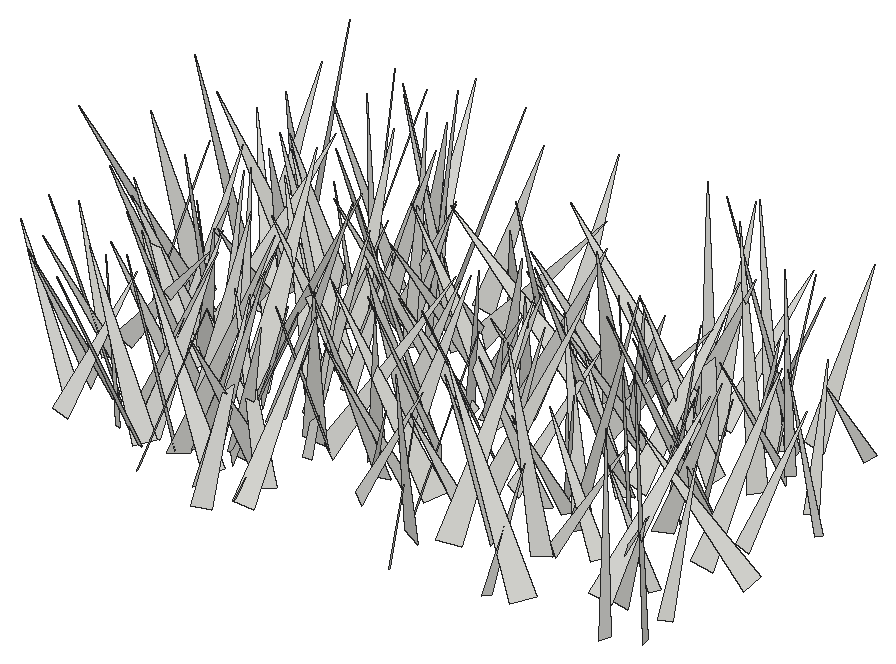
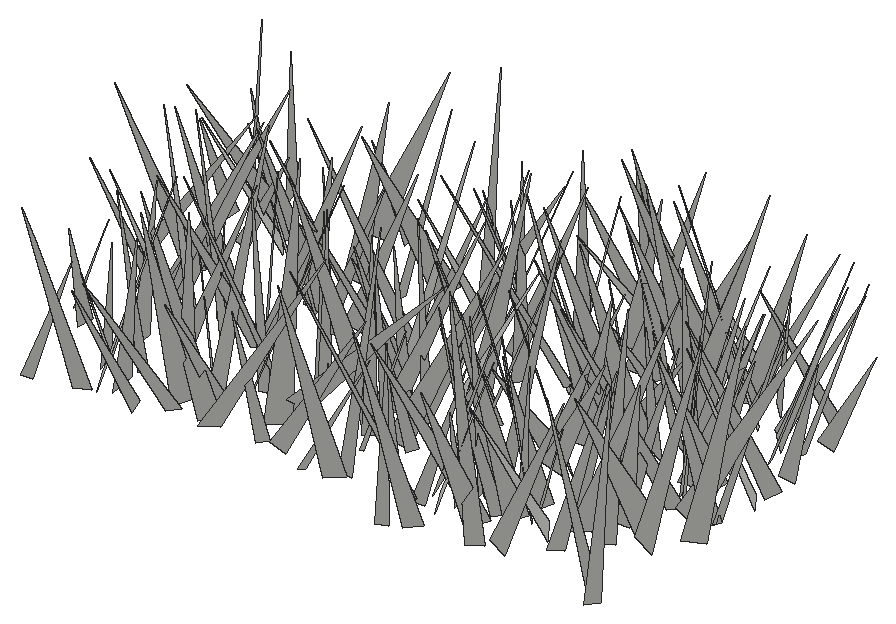
# SketchUp Ruby script. Lengths in inches.
U = 1.inch
M = Sketchup.active_model
def pt(a) = Geom::Point3d.new(a.map { |v| v * U })
def face(e, loops, mat)
  f = e.add_face(loops[0].map { |a| pt(a) })
  loops[1..].each { |l| e.add_face(l.map { |a| pt(a) }).erase! }
  f.material = f.back_material = mat if mat
  f
end
# faces: each face lists its corners as indices into pts; further lists are holes
def faces(e, pts, list, mat = nil) = list.each { |f| face(e, (f[0].is_a?(Array) ? f : [f]).map { |l| l.map { |i| pts[i] } }, mat) }
# xy, xz, yz: faces in a plane at the given z, y or x. An outline is a flat list of corners, or four numbers for a rectangle; further outlines are holes
def ring(l) = l.size == 4 ? [[l[0], l[1]], [l[2], l[1]], [l[2], l[3]], [l[0], l[3]]] : l.each_slice(2).to_a
def flat(e, list, mat, &to3) = list.each { |f| face(e, (f[0].is_a?(Array) ? f : [f]).map { |l| ring(l).map { |u, v| to3.(u, v) } }, mat) }
def xy(e, z, list, mat = nil) = flat(e, list, mat) { |x, y| [x, y, z] }
def xz(e, y, list, mat = nil) = flat(e, list, mat) { |x, z| [x, y, z] }
def yz(e, x, list, mat = nil) = flat(e, list, mat) { |y, z| [x, y, z] }
def lines(e, pts, list) = list.each { |a, b| e.add_line(pt(pts[a]), pt(pts[b])) }
# prism: a flat outline (further loops are holes) pulled along v
def prism(e, loops, v, mat = nil)
  f = face(e, loops, mat); d = Geom::Vector3d.new(v.map { |x| x * U })
  f.pushpull(f.normal.samedirection?(d) ? d.length : -d.length)
end
def box(e, o, s, mat = nil) = prism(e, [[o, [o[0] + s[0], o[1], o[2]], [o[0] + s[0], o[1] + s[1], o[2]], [o[0], o[1] + s[1], o[2]]]], [0, 0, s[2]], mat)
def at(x, y, z, deg = 0) = Geom::Transformation.translation(pt([x, y, z])) * Geom::Transformation.rotation(ORIGIN, Z_AXIS, deg.degrees)
def axes(o, x, y, z) = Geom::Transformation.new([*x, 0, *y, 0, *z, 0, *pt(o).to_a, 1])
def part(name) = M.definitions.add(name)
# library, detail: a bought-in or finely detailed component or shape, given as its bounding box
def library(name, o, s) = part(name).tap { |d| box(d.entities, o, s) }
def detail(e, o, s) = box(e.add_group.entities, o, s)
def put(e, d, t, mat = nil) = e.add_instance(d, t).tap { |i| i.material = mat if mat }
def group(e, t, mat = nil) = e.add_group.tap { |g| g.transformation = t; g.material = mat if mat }.entities
root = M.entities
c1 = part("fur_instance\#9")
p = [[0.8125,0,1.79],[0.67,-0.02,1.48],[0,-0.11,0],[0,0.11,0]]
faces(c1.entities,p,[[0,1,2,3]])
put(root,c1,axes([463.15,234.91,-21.66],[-3.41079,-4.86692,0.40111],[-4.72199,3.16213,-1.78467],[-1.24525,1.33989,5.66881]))
put(root,c1,axes([470.875,231.29,-21.66],[-5.5806,3.5391,0.90465],[3.04631,5.42049,-2.4135],[2.01583,1.60617,6.15169]))
put(root,c1,axes([482.93,236.29,-21.66],[-1.97553,-6.78705,1.45707],[-6.65434,2.28292,1.61176],[1.97656,0.90224,6.88251]))
put(root,c1,axes([470.3,237.66,-21.66],[3.62515,-5.36286,0.15908],[-5.03579,-3.46731,-2.13211],[-1.85105,-1.06996,6.11196]))
put(root,c1,axes([484.31,232.44,-21.66],[2.91558,3.30379,0.88214],[2.68077,-2.92801,2.10571],[-2.12289,0.83996,3.8706]))
put(root,c1,axes([469.28,233.44,-21.66],[7.05742,-1.09775,2.22467],[-1.64487,-7.09246,1.71837],[-1.85705,2.1103,6.93249]))
put(root,c1,axes([493.01,234.44,-21.66],[-4.31341,6.46311,1.11663],[6.32564,3.74609,2.75266],[-1.73345,-2.41229,7.26637]))
put(root,c1,axes([464.99,232.53,-21.66],[4.59925,2.87418,0.36346],[2.61006,-4.40682,1.82035],[-1.25721,1.36572,5.10885]))
put(root,c1,axes([490.875,233.55,-21.66],[4.03542,0.28371,1.50858],[-0.2798,-4.0361,1.5075],[-1.50932,1.50677,3.754]))
put(root,c1,axes([463.28,235.34,-21.66],[-4.72001,4.32069,1.36462],[4.52973,4.45158,1.57294],[-0.11027,-2.07946,6.20264]))
put(root,c1,axes([499.73,233.85,-21.66],[-6.28866,-0.36775,1.68536],[-0.82762,6.23312,-1.72806],[1.51351,1.8804,6.05775]))
put(root,c1,axes([472.62,233.08,-21.66],[-1.93845,6.02083,0.54238],[5.77969,2.01278,-1.68701],[1.77192,0.02133,6.09606]))
put(root,c1,axes([468.76,235.1,-21.66],[-3.29072,5.65648,0.59206],[5.32719,2.82602,2.60955],[-1.99181,-1.7869,6.00123]))
put(root,c1,axes([468.65,237.59,-21.66],[1.7793,-6.50243,0.4842],[-6.28195,-1.575,1.93351],[1.74732,0.95904,6.45825]))
put(root,c1,axes([472.44,235.53,-21.66],[-2.33709,5.71521,1.48586],[5.84354,2.00796,1.46781],[-0.85111,-1.90732,5.99759]))
put(root,c1,axes([468.56,237.07,-21.66],[3.57739,2.98141,0.96801],[3.07785,-3.06266,-1.94177],[0.59384,-2.08684,4.23274]))
put(root,c1,axes([471.87,233.23,-21.66],[4.84887,3.21318,0.05137],[2.84684,-4.33809,2.62966],[-1.49084,2.16682,5.18854]))
put(root,c1,axes([457.1,234.94,-21.66],[0.04423,5.29855,0.55334],[5.02486,0.14232,-1.76445],[1.76963,-0.53655,4.99632]))
put(root,c1,axes([465.27,235.86,-21.66],[-5.24793,-3.08562,0.82091],[-3.15493,4.76816,-2.24651],[-0.49124,2.34081,5.65818]))
put(root,c1,axes([497.93,237.6,-21.66],[1.41621,-4.16021,0.5332],[-4.01988,-1.18575,1.42542],[1.19673,0.94019,4.15706]))
put(root,c1,axes([458.76,238.38,-21.66],[-2.19806,-5.17129,0.07017],[-4.98418,2.09779,-1.52836],[-1.38027,0.66005,5.4072]))
put(root,c1,axes([460.77,235.91,-21.66],[2.36274,4.29484,1.97791],[3.91667,-3.01643,1.87116],[-2.64906,-0.62918,4.53067]))
put(root,c1,axes([501.89,235.02,-21.66],[-7.32928,-2.99407,2.48715],[-3.76161,6.81126,-2.88543],[1.00033,3.67572,7.37273]))
put(root,c1,axes([456.2,239.35,-21.66],[-5.34659,-1.99732,0.9572],[-1.60106,5.21354,1.93576],[1.5304,-1.52357,5.36919]))
put(root,c1,axes([465.65,235.65,-21.66],[7.81962,-2.04899,1.63917],[-2.46618,-7.49875,2.3913],[-0.8962,2.75717,7.72182]))
put(root,c1,axes([462.74,236.34,-21.66],[-0.40245,7.17423,1.83924],[7.10701,0.89237,-1.92572],[2.08393,-1.65784,6.92265]))
put(root,c1,axes([486.96,239.36,-21.66],[-5.96376,-1.66281,1.60864],[-1.32131,6.09893,1.40577],[1.89916,-0.97833,6.02952]))
put(root,c1,axes([460.3,238.46,-21.66],[6.41393,4.45568,0.74677],[4.39818,-5.86174,-2.80093],[1.0328,-2.70854,7.29015]))
put(root,c1,axes([457.24,241.12,-21.66],[-5.6995,-3.45113,0.56108],[-3.05969,5.44221,2.39374],[1.69215,-1.78365,6.21808]))
put(root,c1,axes([477.57,237.99,-21.66],[2.82226,4.09729,0.68802],[3.94816,-2.38599,-1.98631],[1.29353,-1.65697,4.56152]))
put(root,c1,axes([464.25,240.24,-21.66],[-0.98604,-7.77609,1.14314],[-7.75331,0.77346,-1.42635],[-1.28859,1.29646,7.70749]))
put(root,c1,axes([476.89,240.04,-21.66],[4.69242,0.16576,0.10905],[0.19618,-4.2622,-1.96297],[-0.02968,-1.96577,4.26532]))
put(root,c1,axes([455.8,237.6,-21.66],[-1.87407,5.07403,0.37598],[4.58214,1.50899,2.47512],[-2.21159,-1.17322,4.80954]))
put(root,c1,axes([478.56,241.21,-21.66],[-5.31145,-3.30369,0.30508],[-3.10318,5.15062,1.7494],[1.17379,-1.33255,6.00546]))
put(root,c1,axes([495.26,239.72,-21.66],[3.7363,2.07589,0.22504],[1.88074,-3.14536,-2.2112],[0.90706,-2.02911,3.65784]))
put(root,c1,axes([466.17,236.93,-21.66],[6.99612,0.8962,1.32294],[0.53893,-6.91662,1.83548],[-1.5043,1.69005,6.81028]))
put(root,c1,axes([458.17,239.17,-21.66],[-4.54723,-4.75664,0.92618],[-4.80738,4.26788,-1.68375],[-0.61038,1.82216,6.36144]))
put(root,c1,axes([483.75,240.51,-21.66],[-4.12735,0.23871,1.0618],[0.66209,3.85593,1.70672],[0.86374,-1.81501,3.76552]))
put(root,c1,axes([471.13,241.81,-21.66],[1.38948,-7.3294,0.52561],[-7.22169,-1.26322,1.47599],[1.35779,0.7818,7.31247]))
put(root,c1,axes([490.44,239.37,-21.66],[0.55965,-6.1533,3.26603],[-6.71098,-1.35523,-1.40332],[-1.86889,3.02383,6.01722]))
put(root,c1,axes([472.05,241.97,-21.66],[-4.28945,-4.51982,0.83876],[-4.25056,4.33652,1.63064],[1.75072,-0.54543,6.01408]))
put(root,c1,axes([464.37,239.22,-21.66],[-0.74897,7.24815,2.93985],[7.55595,1.43371,-1.60981],[2.0214,-2.6736,7.1067]))
put(root,c1,axes([501.15,237.84,-21.66],[-4.3486,2.21974,0.80785],[1.83051,4.23636,-1.78683],[1.49303,1.27131,4.54366]))
put(root,c1,axes([477.14,240.85,-21.66],[-2.01567,-6.30283,1.43527],[-6.28052,1.55369,-1.99742],[-1.52993,1.92587,6.30864]))
put(root,c1,axes([498.44,240.22,-21.66],[-0.27177,-3.75184,1.87256],[-3.70908,-0.66019,-1.86105],[-1.95589,1.77327,3.26904]))
put(root,c1,axes([462.15,241.86,-21.66],[-4.28655,1.17606,1.86698],[1.8295,4.17484,1.57066],[1.23356,-2.10497,4.15821]))
put(root,c1,axes([481.04,240.95,-21.66],[-4.16636,5.9481,1.52453],[5.74666,3.12806,3.50054],[-2.16332,-3.14611,6.36276]))
put(root,c1,axes([496.4375,237.5,-21.66],[-2.65177,6.66161,0.65253],[5.97681,2.67255,-2.995],[3.01341,0.56142,6.51452]))
put(root,c1,axes([490.56,240.375,-21.66],[2.95433,4.07724,0.35212],[3.82019,-2.59183,-2.04072],[1.46767,-1.46099,4.60298]))
put(root,c1,axes([485.14,237.13,-21.66],[-5.76444,5.45156,1.05869],[4.71185,5.60881,-3.22628],[2.93919,1.70025,7.24841]))
put(root,c1,axes([475,242.86,-21.66],[6.59264,-0.88288,1.14982],[-0.53637,-6.4595,-1.88457],[-1.3468,-1.74924,6.37893]))
put(root,c1,axes([481.52,238.15,-21.66],[4.88269,3.53574,0.69101],[3.04894,-4.67553,2.3797],[-1.91908,1.56767,5.53887]))
put(root,c1,axes([467.67,238.9,-21.66],[3.89032,1.8987,0.46131],[1.51623,-3.58179,1.95558],[-1.23244,1.58688,3.86204]))
put(root,c1,axes([493.38,241.23,-21.66],[-3.16425,3.77948,0.90882],[3.82647,2.82214,1.58634],[-0.68447,-1.69527,4.66695]))
put(root,c1,axes([467.05,241.04,-21.66],[-1.66623,3.3763,0.05798],[2.90925,1.40249,1.93607],[-1.71436,-0.9015,3.22914]))
put(root,c1,axes([496.47,238.77,-21.66],[4.76717,4.34009,0.09976],[4.0907,-4.54047,2.05487],[-1.45344,1.45601,6.11063]))
put(root,c1,axes([458.59,243.71,-21.66],[0.69444,-4.60057,1.02449],[-4.36557,-1.0182,-1.61314],[-1.77671,0.70364,4.36409]))
put(root,c1,axes([488.49,244.5,-21.66],[1.56687,-4.2825,0.24372],[-4.04586,-1.5617,-1.43053],[-1.42486,-0.27491,4.32996]))
put(root,c1,axes([472.04,239.95,-21.66],[2.45384,5.3856,0.3895],[5.06414,-2.44383,1.88676],[-1.87372,0.44803,5.60947]))
put(root,c1,axes([478,245.25,-21.66],[-5.39374,-4.42373,0.73063],[-4.15874,5.36317,1.77113],[1.67573,-0.92879,6.74722]))
put(root,c1,axes([465.64,243.59,-21.66],[3.73133,2.74864,1.27928],[3.02044,-3.19509,-1.94493],[0.26177,-2.31318,4.20655]))
put(root,c1,axes([455.11,242.2,-21.66],[-1.60239,4.56784,1.22355],[4.62571,1.24567,1.40748],[-0.98238,-1.58525,4.63161]))
put(root,c1,axes([486.93,243.97,-21.66],[0.61294,-5.47928,1.38132],[-5.30961,-1.0339,-1.7451],[-1.93355,1.10218,5.22999]))
put(root,c1,axes([502.45,244.53,-21.66],[-5.96221,1.49508,0.02596],[1.36332,5.39133,2.61894],[-0.61423,-2.54602,5.56097]))
put(root,c1,axes([472.27,241.57,-21.66],[3.56611,7.00423,0.23479],[6.50816,-3.2121,-3.02618],[2.59966,-1.56674,7.25387]))
put(root,c1,axes([460,242.77,-21.66],[-2.19401,4.08598,0.64459],[3.98986,1.89782,1.55038],[-1.09165,-1.27572,4.37096]))
put(root,c1,axes([480.73,246.9375,-21.66],[-3.5223,-6.70382,0.02091],[-6.50166,3.42181,1.83516],[1.63401,-0.83562,7.34711]))
put(root,c1,axes([454.53,244.24,-21.66],[2.58062,-5.27777,0.62862],[-4.46822,-1.77579,3.43383],[2.87837,1.97518,4.76689]))
put(root,c1,axes([459.5,245.66,-21.66],[6.23542,-1.61716,0.46655],[-1.48447,-6.12774,-1.40019],[-0.79324,-1.24458,6.2877]))
put(root,c1,axes([475.46,246.4,-21.66],[5.45366,-4.66647,1.60556],[-4.21255,-5.64853,-2.10822],[-2.57063,-0.64365,6.86103]))
put(root,c1,axes([459.94,244.1875,-21.66],[-5.34119,3.3335,0.99515],[3.47843,5.14626,1.43085],[0.05516,-1.74201,6.13133]))
put(root,c1,axes([469.27,243.625,-21.66],[2.86437,6.58912,2.04567],[6.83224,-2.40073,-1.83379],[0.96006,-2.57407,6.94682]))
put(root,c1,axes([467.7,242.38,-21.66],[7.57177,-0.43303,1.80554],[-0.88332,-7.50835,1.90355],[-1.63317,2.05334,7.34137]))
put(root,c1,axes([487.44,245.54,-21.66],[4.97524,0.71585,1.07536],[1.04452,-4.74693,-1.67259],[-0.76015,-1.83742,4.74004]))
put(root,c1,axes([483.26,243.14,-21.66],[2.59444,7.48207,1.23534],[7.31718,-2.12705,-2.48457],[1.99156,-1.93206,7.51927]))
put(root,c1,axes([459.28,246.41,-21.66],[3.15853,-4.87453,2.05329],[-4.28659,-3.76007,-2.33247],[-3.09874,0.23284,5.31949]))
put(root,c1,axes([490.16,243.68,-21.66],[-1.21025,6.4146,1.42422],[6.45546,0.89059,1.47445],[-1.22575,-1.64315,6.35907]))
put(root,c1,axes([490.11,242.9375,-21.66],[7.12046,1.58475,2.39098],[0.70942,-7.17277,2.64146],[-2.77938,2.22916,6.79964]))
put(root,c1,axes([497.89,247.15,-21.66],[-2.49506,-7.82927,1.12782],[-7.54738,2.00233,-2.79687],[-2.3678,1.86761,7.7266]))
put(root,c1,axes([459.04,247.32,-21.66],[6.14406,2.36607,3.59044],[3.36505,-6.54408,-1.44586],[-2.67694,-2.79567,6.42319]))
put(root,c1,axes([484.18,244.47,-21.66],[1.81357,5.35205,0.20733],[5.12174,-1.66889,-1.72019],[1.56691,-0.73948,5.38279]))
put(root,c1,axes([462.77,242.97,-21.66],[1.87355,6.48838,0.26131],[6.01197,-1.83596,2.48253],[-2.45429,0.45575,6.28063]))
put(root,c1,axes([498.75,244.36,-21.66],[-0.63507,6.95916,1.46669],[6.78735,1.03289,-1.962],[2.12438,-1.21968,6.70699]))
put(root,c1,axes([494.3,246.16,-21.66],[5.13759,-3.83835,0.8309],[-3.9202,-4.93031,1.46363],[0.23526,1.66651,6.24384]))
put(root,c1,axes([498.59,247,-21.66],[-4.44374,-5.75342,0.61079],[-5.6055,4.0905,-2.25122],[-1.43294,1.84058,6.91236]))
put(root,c1,axes([455.02,248.97,-21.66],[-6.16239,-2.08969,1.53365],[-1.42213,6.03269,2.50561],[2.16712,-1.98337,6.00531]))
put(root,c1,axes([464.27,244.57,-21.66],[-3.17908,7.18759,1.82609],[7.05927,3.54175,-1.65087],[2.27218,-0.9472,7.68392]))
put(root,c1,axes([475.26,245.8,-21.66],[0.44188,5.84269,1.52194],[5.83939,-0.02571,-1.59672],[1.53457,-1.58458,5.63763]))
put(root,c1,axes([493.96,248.1,-21.66],[-2.04339,-2.88899,0.9747],[-2.5158,2.26047,1.42575],[1.7225,-0.12566,3.23866]))
put(root,c1,axes([489.81,248.31,-21.66],[-2.55131,-7.67351,1.38924],[-7.65133,2.18082,-2.00574],[-1.50657,1.91917,7.83383]))
put(root,c1,axes([463.2,244.71,-21.66],[1.09357,6.43106,0.77169],[6.11568,-1.28298,2.02542],[-2.13365,-0.38127,6.20097]))
put(root,c1,axes([482.73,245.125,-21.66],[-4.41851,1.16155,1.66424],[0.34777,4.36157,-2.12081],[1.99949,1.8082,4.04655]))
put(root,c1,axes([463.74,246.08,-21.66],[7.28902,-0.71217,0.57332],[-0.83779,-7.04721,1.89755],[-0.36604,1.94818,7.07364]))
put(root,c1,axes([456.89,249.64,-21.66],[-1.39061,-8.04384,0.83594],[-7.45661,0.94696,-3.29214],[-3.13068,1.31752,7.46987]))
put(root,c1,axes([457.53,249.09,-21.66],[-3.39488,-3.98848,1.56761],[-3.7052,3.73666,1.48306],[2.15333,0.14147,5.02331]))
put(root,c1,axes([476.7,246.29,-21.66],[-6.97142,-3.26118,0.0354],[-2.96258,6.29742,-3.28677],[-1.3637,2.99072,6.9594]))
put(root,c1,axes([468.02,249.14,-21.66],[-6.07615,0.58264,0.90457],[0.83184,5.83413,1.82981],[0.68247,-1.92372,5.8233]))
put(root,c1,axes([467.43,246.55,-21.66],[-3.01404,5.97197,0.86388],[5.95256,2.78442,1.51964],[-0.98886,-1.44144,6.51457]))
put(root,c1,axes([494.42,249.86,-21.66],[6.71484,1.18998,0.43364],[1.2609,-6.06064,-2.89345],[0.11927,-2.92333,6.1752]))
put(root,c1,axes([454.84,245.55,-21.66],[5.18703,3.91751,0.7095],[3.72248,-5.18551,1.41748],[-1.41191,0.72053,6.34373]))
put(root,c1,axes([491.78,246.1,-21.66],[-6.04222,-2.58238,2.07365],[-3.21518,5.60869,-2.38377],[0.79453,3.05796,6.1233]))
put(root,c1,axes([476.49,250.1875,-21.66],[-4.86866,0.51762,1.11395],[0.97098,4.41082,2.19421],[0.75234,-2.34296,4.3769]))
put(root,c1,axes([472.82,248.13,-21.66],[2.29321,-4.71361,1.70331],[-4.8602,-1.63403,2.02152],[1.22385,2.34308,4.83635]))
put(root,c1,axes([457.65,245.64,-21.66],[-5.19171,3.73852,1.55221],[3.028,5.26206,-2.54592],[2.68647,1.29382,5.8693]))
put(root,c1,axes([477.86,250.1,-21.66],[0.93957,-4.99379,0.05949],[-4.70596,-0.86502,1.71172],[1.67197,0.37157,4.78443]))
put(root,c1,axes([489.8,248.01,-21.66],[-1.66543,4.2087,0.7623],[4.0491,1.28782,1.73616],[-1.37806,-1.30242,4.18002]))
put(root,c1,axes([484.14,250.51,-21.66],[-0.53016,-5.209,0.61736],[-4.97847,0.69512,1.58982],[1.65216,0.4231,4.98871]))
put(root,c1,axes([455.08,249.32,-21.66],[2.87453,-4.20489,0.68169],[-4.14129,-2.56592,1.63539],[0.99777,1.46412,4.82385]))
put(root,c1,axes([499.25,247.58,-21.66],[0.30593,5.01742,0.69432],[4.86404,-0.09691,-1.44288],[1.4134,-0.75252,4.8152]))
put(root,c1,axes([476.16,250.31,-21.66],[6.10646,0.88523,1.50787],[1.27518,-6.00248,-1.64024],[-1.19633,-1.87958,5.94829]))
put(root,c1,axes([483.65,250.78,-21.66],[5.31663,-1.02418,0.76649],[-0.77202,-5.18142,-1.56841],[-1.02002,-1.41668,5.18224]))
put(root,c1,axes([491.88,250.05,-21.66],[6.71325,2.37054,1.67819],[2.73448,-6.58312,-1.63968],[-0.97898,-2.13225,6.9281]))
put(root,c1,axes([459.37,252.73,-21.66],[4.70734,-3.12135,0.14145],[-2.64852,-4.12178,-2.81392],[-1.65776,-2.27815,4.89732]))
put(root,c1,axes([478.77,250.58,-21.66],[-7.28796,2.50197,0.93453],[2.66483,6.99355,2.0583],[0.17855,-2.25345,7.42547]))
put(root,c1,axes([465.61,249.68,-21.66],[4.35224,4.23695,0.82253],[4.28263,-4.09432,-1.57033],[0.53605,-1.68972,5.86752]))
put(root,c1,axes([454.67,251.65,-21.66],[4.91943,-4.73173,2.30235],[-4.40019,-5.42749,-1.75256],[-2.8859,0.2095,6.59686]))
put(root,c1,axes([476.04,253.34,-21.66],[2.18391,-6.70079,0.42323],[-6.08063,-2.16263,-2.86325],[-2.84706,-0.52116,6.43986]))
put(root,c1,axes([477.76,250.08,-21.66],[2.95683,-4.48742,1.40063],[-4.613,-2.45121,1.88504],[0.90496,2.16707,5.03253]))
put(root,c1,axes([486.67,253.97,-21.66],[-5.64756,-4.03637,0.24701],[-3.60758,5.22048,2.82493],[1.82721,-2.16853,6.3409]))
put(root,c1,axes([470.7,253.74,-21.66],[-6.78403,-3.28205,0.63683],[-2.89291,6.48484,2.60352],[1.67585,-2.09175,7.07224]))
put(root,c1,axes([488.67,254.82,-21.66],[-2.64275,-7.72517,0.10148],[-7.35563,2.5487,2.46402],[2.36287,-0.70608,7.78402]))
put(root,c1,axes([468.89,247.77,-21.66],[-4.90566,2.32822,0.51514],[1.6552,4.17303,-3.098],[1.71648,2.62995,4.45965]))
put(root,c1,axes([458,249.18,-21.66],[0.84349,7.5995,0.98427],[7.14395,-0.42161,-2.86687],[2.77222,-1.22577,7.08837]))
put(root,c1,axes([477.97,253.5625,-21.66],[0.06322,-6.05576,0.15688],[-5.74231,-0.00994,1.93043],[1.92942,0.16885,5.74018]))
put(root,c1,axes([496.73,249.05,-21.66],[5.00084,3.55671,0.83126],[3.26277,-4.98345,1.69387],[-1.6418,0.92989,5.89825]))
put(root,c1,axes([466.95,249.97,-21.66],[-1.95645,6.57203,0.15793],[5.85701,1.66776,3.15567],[-2.98529,-1.03499,6.08778]))
put(root,c1,axes([478.7,252.13,-21.66],[4.47531,-6.51665,1.20055],[-6.35255,-3.80729,3.0143],[1.88498,2.64087,7.30815]))
put(root,c1,axes([492.91,252.92,-21.66],[-6.35837,1.48,1.02188],[1.69793,6.17763,1.61781],[0.593,-1.81932,6.3247]))
put(root,c1,axes([489.7,249.34,-21.66],[0.36828,7.38641,0.21711],[7.15433,-0.30198,-1.86176],[1.84979,-0.30261,7.15741]))
put(root,c1,axes([486.15,253.39,-21.66],[-1.36067,-5.7583,1.83351],[-5.61411,1.9,1.80082],[2.23642,1.26617,5.63617]))
put(root,c1,axes([466.64,255.35,-21.66],[-3.41876,-7.6362,0.72671],[-7.48826,3.49493,1.49637],[1.66304,0.03883,8.23167]))
put(root,c1,axes([490.25,253.27,-21.66],[3.23905,1.92957,1.10614],[2.22288,-2.8741,-1.49551],[-0.07469,-1.85863,3.46094]))
put(root,c1,axes([474.83,253.43,-21.66],[1.43751,-4.12245,0.23292],[-3.7226,-1.18725,1.96162],[1.78636,0.84328,3.90039]))
put(root,c1,axes([460.84,254.85,-21.66],[-7.92224,1.63819,2.17065],[2.33717,7.51957,2.85498],[1.39032,-3.306,7.56932]))
put(root,c1,axes([458.68,255.1875,-21.66],[6.56004,-2.8558,0.90961],[-2.50702,-6.42798,-2.10074],[-1.6425,-1.59457,6.83935]))
put(root,c1,axes([483.9,253.9,-21.66],[5.26826,5.58359,0.80335],[4.69893,-3.73546,-4.8521],[3.1212,-3.80083,5.9488]))
put(root,c1,axes([465.9,252.64,-21.66],[4.67492,4.49227,1.13099],[4.6277,-4.45606,-1.42912],[0.20972,-1.8104,6.324]))
put(root,c1,axes([483.08,255.92,-21.66],[6.31463,-5.10403,0.36931],[-4.97216,-6.25818,-1.47472],[-1.21044,-0.91981,7.98441]))
put(root,c1,axes([460.55,251,-21.66],[-2.20757,6.36235,0.08993],[6.1827,2.12231,1.62203],[-1.50393,-0.61421,6.5362]))
put(root,c1,axes([501.91,251.62,-21.66],[-5.07583,-0.99149,0.0646],[-0.93064,4.62637,-2.11704],[-0.34804,2.08923,4.7186]))
put(root,c1,axes([495.84,256.04,-21.66],[-4.51609,-3.87484,0.43498],[-3.47065,4.29803,2.25393],[1.77713,-1.453,5.5072]))
put(root,c1,axes([477.19,255.29,-21.66],[-3.37323,-1.69913,0.74168],[-1.13548,3.11072,1.96213],[1.46554,-1.50074,3.22735]))
put(root,c1,axes([456.77,253.86,-21.66],[-2.69995,-7.06667,2.40673],[-7.39529,2.18224,-1.88876],[-1.01973,2.88442,7.32531]))
put(root,c1,axes([474.93,255.34,-21.66],[0.27487,-5.90315,0.86813],[-5.62576,0.03312,2.00651],[1.98787,0.91,5.55848]))
put(root,c1,axes([483.4,254.73,-21.66],[-5.86481,5.71927,0.12396],[4.62698,4.63811,4.91939],[-3.36399,-3.59156,6.55024]))
put(root,c1,axes([461.88,254.39,-21.66],[-1.46223,5.38545,2.28823],[5.73287,0.84616,1.67196],[-1.17188,-2.58033,5.32407]))
put(root,c1,axes([493.32,256.08,-21.66],[-0.9776,-5.25666,1.94415],[-5.10339,1.65068,1.89699],[2.31681,1.41798,4.99896]))
put(root,c1,axes([499.82,253.48,-21.66],[-4.30895,1.90574,0.59057],[1.67064,4.21479,-1.41144],[1.09067,1.07302,4.49519]))
put(root,c1,axes([467.54,255.27,-21.66],[3.43659,4.37627,1.35344],[4.55407,-3.08156,-1.59944],[0.49399,-2.03617,5.32951]))
put(root,c1,axes([464.3125,254.35,-21.66],[-4.28089,-1.18354,0.47624],[-1.27514,3.91753,-1.72642],[-0.03977,1.79046,4.09221]))
put(root,c1,axes([476.07,258.25,-21.66],[-2.59583,-7.17613,0.91864],[-6.91744,2.74775,1.9178],[2.11891,0.17907,7.38629]))
put(root,c1,axes([495.76,253.38,-21.66],[-8.22184,1.12863,0.67504],[0.91948,7.98903,-2.15825],[0.94024,2.05661,8.01339]))
put(root,c1,axes([465.83,256.42,-21.66],[0.54416,-5.67013,1.84078],[-5.27926,0.40028,2.79359],[2.76917,1.87733,4.9641]))
put(root,c1,axes([470.54,258.22,-21.66],[3.27584,-2.78093,0.2499],[-2.38988,-2.99185,-1.96583],[-1.44378,-1.35736,3.82103]))
put(root,c1,axes([464.33,254,-21.66],[-4.85985,3.92503,1.53679],[3.59209,5.08366,-1.6245],[2.20555,0.36911,6.032]))
put(root,c1,axes([468.42,254.28,-21.66],[-7.01527,0.64484,2.20419],[0.06996,7.14138,-1.86657],[2.29551,1.75305,6.79307]))
put(root,c1,axes([457.87,252.04,-21.66],[-6.65412,4.03174,0.74119],[3.28122,6.08544,-3.64454],[2.45722,2.79179,6.87384]))
put(root,c1,axes([464.7,256.12,-21.66],[5.22316,-4.20753,1.34718],[-4.41725,-5.01042,1.47756],[-0.07792,1.998,6.54228]))
put(root,c1,axes([460.52,257.55,-21.66],[-5.0365,1.95588,2.0654],[2.56555,4.93734,1.5806],[1.22852,-2.29236,5.16658]))
put(root,c1,axes([481.3125,258.21,-21.66],[0.83306,-5.07313,1.39633],[-4.3947,-1.44829,-2.63999],[-2.89363,0.73905,4.41148]))
put(root,c1,axes([469.78,254.1,-21.66],[4.59054,6.55576,1.84003],[6.00661,-4.94402,2.62946],[-3.20693,0.124,7.5589]))
put(root,c1,axes([486.77,257.875,-21.66],[2.93254,-6.52755,1.0505],[-6.19008,-2.30697,2.94501],[2.32281,2.09313,6.52193]))
put(root,c1,axes([464.77,255.55,-21.66],[-6.75602,-0.97126,1.58692],[-1.43223,6.52998,-2.10085],[1.1876,2.34979,6.49412]))
put(root,c1,axes([464.48,255.01,-21.66],[5.18637,5.57386,2.23152],[5.04396,-5.64447,2.37581],[-3.2567,0.13438,7.23339]))
put(root,c1,axes([470.87,255.74,-21.66],[-7.866,-1.33504,0.19154],[-1.32695,7.45779,-2.51268],[-0.24134,2.50839,7.5725]))
put(root,c1,axes([486.14,258.7,-21.66],[-7.10232,2.48969,0.17848],[2.39972,6.66255,2.55443],[-0.68683,-2.46683,7.07929]))
put(root,c1,axes([482.45,258.19,-21.66],[1.69765,-3.69471,0.41656],[-3.54176,-1.46758,1.41724],[1.13153,0.9496,3.81108]))
put(root,c1,axes([470.97,258.11,-21.66],[5.03462,6.0848,0.40692],[5.07887,-3.8915,-4.64748],[3.37572,-3.22012,6.38538]))
put(root,c1,axes([478.5625,259.28,-21.66],[-4.09373,-0.36711,0.23804],[-0.24891,3.79616,1.57392],[0.35983,-1.55061,3.79686]))
put(root,c1,axes([490.3,255.63,-21.66],[1.13757,8.04859,1.54719],[7.76789,-1.55698,2.3882],[-2.61411,-1.12413,7.76984]))
put(root,c1,axes([487.18,256.16,-21.66],[-2.89965,3.32427,1.06428],[2.78447,3.03733,-1.90073],[2.1048,0.5615,3.98069]))
put(root,c1,axes([496,256.26,-21.66],[-6.18556,-0.57175,1.0735],[-0.94708,5.75521,-2.39186],[0.76312,2.5082,5.73298]))
put(root,c1,axes([468.7,256.52,-21.66],[-4.6642,0.46344,0.8289],[0.1067,4.38406,-1.85075],[0.94364,1.79496,4.30631]))
put(root,c1,axes([464.67,260.14,-21.66],[0.15208,-7.64456,1.76209],[-7.47072,0.39677,2.36609],[2.3943,1.72356,7.27077]))
put(root,c1,axes([494.63,258.58,-21.66],[-7.44301,-3.63877,0.95843],[-3.76282,7.20814,-1.85509],[0.01898,2.08796,8.0745]))
put(root,c1,axes([469.61,257.49,-21.66],[-7.1733,-2.93015,0.73361],[-2.97558,6.52972,-3.01478],[-0.51951,3.05896,7.13815]))
put(root,c1,axes([498.42,260.85,-21.66],[2.63611,-2.6678,0.56163],[-2.26437,-2.5776,-1.61563],[-1.51829,-0.78771,3.38467]))
put(root,c1,axes([489.14,257.29,-21.66],[-5.55671,4.70477,2.20019],[4.40361,5.97611,-1.65743],[2.7539,-0.06297,7.08977]))
put(root,c1,axes([470.57,261.62,-21.66],[5.43533,-0.93824,0.08866],[-0.80913,-4.91198,-2.3767],[-0.48317,-2.32876,4.97739]))
put(root,c1,axes([454.73,261.3125,-21.66],[6.40589,-1.32849,1.4611],[-0.83624,-6.31798,-2.07823],[-1.78897,-1.80373,6.20333]))
put(root,c1,axes([463.44,259.51,-21.66],[-0.2537,5.53184,2.90433],[5.7111,-0.97344,2.35297],[-2.53371,-2.74807,5.0129]))
put(root,c1,axes([469.34,255.4375,-21.66],[6.78257,3.66457,1.14232],[2.83952,-6.35069,3.51329],[-2.58286,2.6414,6.86216]))
put(root,c1,axes([462.27,256.08,-21.66],[5.32818,4.49942,0.50618],[3.89144,-4.95023,3.04014],[-2.31467,2.03493,6.2763]))
put(root,c1,axes([493.37,257.98,-21.66],[-7.58228,1.17889,0.51367],[1.00041,7.33787,-2.07353],[0.80796,1.97752,7.38791]))
put(root,c1,axes([476.41,258.86,-21.66],[-2.09917,6.50868,2.06271],[6.47308,2.58358,-1.56477],[2.17184,-1.40938,6.65739]))
put(root,c1,axes([493.51,258.04,-21.66],[3.73526,4.02595,0.93613],[3.5763,-3.78049,1.98866],[-2.07237,0.73241,5.11915]))
put(root,c1,axes([489.04,258.48,-21.66],[-0.72981,5.66267,0.18679],[5.27184,0.7477,-2.06932],[2.0757,0.09199,5.32132]))
put(root,c1,axes([468.97,260.61,-21.66],[2.35297,-5.60644,2.50548],[-6.03434,-1.6135,2.05656],[1.13856,3.03489,5.72182]))
put(root,c1,axes([494.92,259.89,-21.66],[0.03903,6.40601,1.64221],[6.43648,0.34027,-1.48032],[1.51842,-1.60705,6.23275]))
put(root,c1,axes([491.09,259.58,-21.66],[4.64309,0.99306,0.50279],[0.80416,-4.48393,1.43003],[-0.7696,1.30595,4.52764]))
put(root,c1,axes([456.37,259.38,-21.66],[6.51752,3.06728,2.32468],[2.5593,-6.86862,1.88745],[-2.87443,0.8392,6.95153]))
put(root,c1,axes([466.09,258.05,-21.66],[-5.16112,5.15909,0.10388],[4.87926,4.92701,-2.27629],[1.67923,1.54029,6.93338]))
